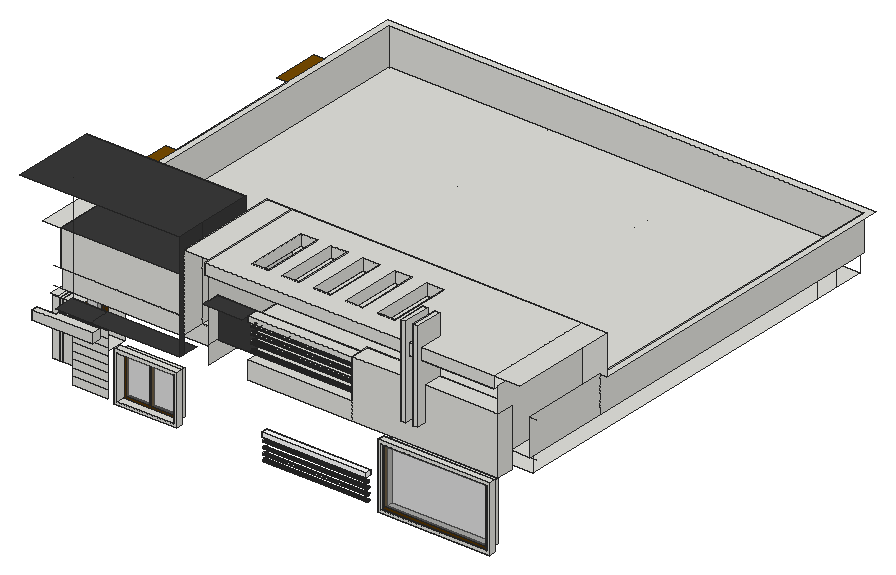
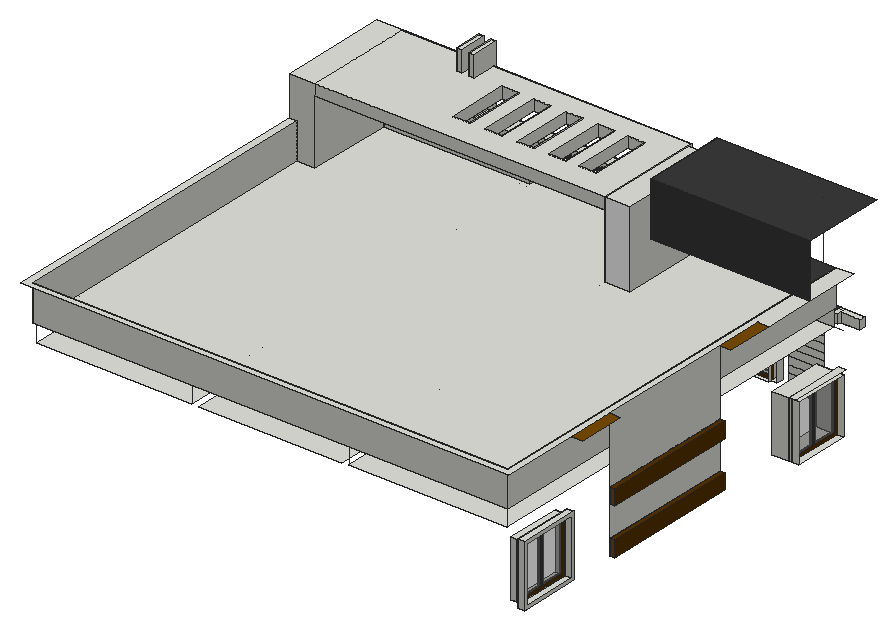
# SketchUp Ruby script. Lengths in inches.
U = 1.inch
M = Sketchup.active_model
def pt(a) = Geom::Point3d.new(a.map { |v| v * U })
def face(e, loops, mat)
  f = e.add_face(loops[0].map { |a| pt(a) })
  loops[1..].each { |l| e.add_face(l.map { |a| pt(a) }).erase! }
  f.material = f.back_material = mat if mat
  f
end
# faces: each face lists its corners as indices into pts; further lists are holes
def faces(e, pts, list, mat = nil) = list.each { |f| face(e, (f[0].is_a?(Array) ? f : [f]).map { |l| l.map { |i| pts[i] } }, mat) }
# xy, xz, yz: faces in a plane at the given z, y or x. An outline is a flat list of corners, or four numbers for a rectangle; further outlines are holes
def ring(l) = l.size == 4 ? [[l[0], l[1]], [l[2], l[1]], [l[2], l[3]], [l[0], l[3]]] : l.each_slice(2).to_a
def flat(e, list, mat, &to3) = list.each { |f| face(e, (f[0].is_a?(Array) ? f : [f]).map { |l| ring(l).map { |u, v| to3.(u, v) } }, mat) }
def xy(e, z, list, mat = nil) = flat(e, list, mat) { |x, y| [x, y, z] }
def xz(e, y, list, mat = nil) = flat(e, list, mat) { |x, z| [x, y, z] }
def yz(e, x, list, mat = nil) = flat(e, list, mat) { |y, z| [x, y, z] }
def lines(e, pts, list) = list.each { |a, b| e.add_line(pt(pts[a]), pt(pts[b])) }
# prism: a flat outline (further loops are holes) pulled along v
def prism(e, loops, v, mat = nil)
  f = face(e, loops, mat); d = Geom::Vector3d.new(v.map { |x| x * U })
  f.pushpull(f.normal.samedirection?(d) ? d.length : -d.length)
end
def box(e, o, s, mat = nil) = prism(e, [[o, [o[0] + s[0], o[1], o[2]], [o[0] + s[0], o[1] + s[1], o[2]], [o[0], o[1] + s[1], o[2]]]], [0, 0, s[2]], mat)
def at(x, y, z, deg = 0) = Geom::Transformation.translation(pt([x, y, z])) * Geom::Transformation.rotation(ORIGIN, Z_AXIS, deg.degrees)
def axes(o, x, y, z) = Geom::Transformation.new([*x, 0, *y, 0, *z, 0, *pt(o).to_a, 1])
def part(name) = M.definitions.add(name)
# library, detail: a bought-in or finely detailed component or shape, given as its bounding box
def library(name, o, s) = part(name).tap { |d| box(d.entities, o, s) }
def detail(e, o, s) = box(e.add_group.entities, o, s)
def put(e, d, t, mat = nil) = e.add_instance(d, t).tap { |i| i.material = mat if mat }
def group(e, t, mat = nil) = e.add_group.tap { |g| g.transformation = t; g.material = mat if mat }.entities
root = M.entities
M.materials.add("[Color C07]").color = [120, 76, 0]
M.materials.add("[Color C08]").color = [85, 51, 0]
M.materials.add("[Color M00]").color = [255, 255, 255]
M.materials.add("[Color M07]").color = [58, 58, 58]
M.materials.add("[Translucent Glass Gray]").color = [128, 128, 128]
M.materials["[Translucent Glass Gray]"].alpha = 0.5
M.materials.add("[Wood Veneer 01]1").color = [120, 70, 37]
c1 = part("Group\#4")
xy(c1.entities,0,[[0,0,0.4375,8.25]],"[Color C08]")
xy(c1.entities,9.875,[[0,0,0.4375,8.25]],"[Color C08]")
xz(c1.entities,0,[[0,0,0.4375,9.875]],"[Color C08]")
xz(c1.entities,0.45,[[0,0.45,0.4375,9.42]],"[Color C08]")
xz(c1.entities,4.05,[[0,0.49,0.4375,9.45]],"[Color C08]")
xz(c1.entities,4.38,[[0,0.49,0.4375,9.45]],"[Color C08]")
xz(c1.entities,7.8,[[0,0.45,0.4375,9.42]],"[Color C08]")
xz(c1.entities,8.25,[[0,0,0.4375,9.875]],"[Color C08]")
yz(c1.entities,0,[[[0,0,8.25,9.875],[0.45,0.45,4.05,0.49,4.05,9.45,0.45,9.42],[7.8,0.45,7.8,9.42,4.38,9.45,4.38,0.49]]],"[Color C08]")
yz(c1.entities,0,[[0.45,0.45,0.45,9.42,4.05,9.45,4.05,0.49],[7.8,0.45,4.38,0.49,4.38,9.45,7.8,9.42]],"[Translucent Glass Gray]")
yz(c1.entities,0.4375,[[[0,0,8.25,9.875],[0.45,0.45,0.45,9.42,4.05,9.45,4.05,0.49],[7.8,0.45,4.38,0.49,4.38,9.45,7.8,9.42]]],"[Color C08]")
p = [[0,4.05,0.49],[0,0.45,0.45],[0.4375,0.45,0.45],[0.4375,4.05,0.49],[0,7.8,0.45],[0,4.38,0.49],
  [0.4375,4.38,0.49],[0.4375,7.8,0.45],[0,0.45,9.42],[0,4.05,9.45],[0.4375,4.05,9.45],[0.4375,0.45,9.42],
  [0,4.38,9.45],[0,7.8,9.42],[0.4375,7.8,9.42],[0.4375,4.38,9.45]]
faces(c1.entities,p,[[0,1,2,3],[4,5,6,7],[8,9,10,11],[12,13,14,15]],"[Color C08]")
c2 = part("Group\#3")
xy(c2.entities,0,[[0,0,69.125,3.25]],"[Color C08]")
xy(c2.entities,1.72,[[1.72,0,67.41,3.25]],"[Color C08]")
xy(c2.entities,48.28,[[1.72,0,67.41,3.25]],"[Color C08]")
xy(c2.entities,50,[[0,0,69.125,3.25]],"[Color C08]")
xz(c2.entities,0,[[[0,0,69.125,50],[1.72,1.72,67.41,48.28]]],"[Color C08]")
xz(c2.entities,0,[[1.72,1.72,67.41,48.28]],"[Translucent Glass Gray]")
xz(c2.entities,3.25,[[[0,0,69.125,50],[1.72,1.72,67.41,48.28]]],"[Color C08]")
yz(c2.entities,0,[[0,0,3.25,50]],"[Color C08]")
yz(c2.entities,1.72,[[0,1.72,3.25,48.28]],"[Color C08]")
yz(c2.entities,67.41,[[0,1.72,3.25,48.28]],"[Color C08]")
yz(c2.entities,69.125,[[0,0,3.25,50]],"[Color C08]")
prism(root,[[[70.87,180.75,670.36],[95.94,180.75,670.36],[95.94,185.5,670.36],[151.38,185.5,670.36],[151.38,172.6875,670.36],[70.87,172.6875,670.36]]],[0,0,12.45])
prism(root,[[[347.125,192.875,732.3],[347.125,193.13,732.92],[347.125,193.54,733.45],[347.125,194.07,733.86],[347.125,194.6875,734.12],[347.125,195.35,734.2],[347.125,196.01,734.12],[347.125,196.63,733.86],[347.125,197.16,733.45],[347.125,197.57,732.92],[347.125,197.83,732.3],[347.125,197.91,731.64],[347.125,197.83,730.98],[347.125,197.57,730.36],[347.125,197.16,729.83],[347.125,196.63,729.42],[347.125,196.01,729.17],[347.125,195.35,729.08],[347.125,194.6875,729.17],[347.125,194.07,729.42],[347.125,193.54,729.83],[347.125,193.13,730.36],[347.125,192.875,730.98],[347.125,192.79,731.64]]],[138.875,0,0])
xy(root,581.63,[[39.625,246.5625,48.625,321.8125],[48.625,246.5625,75,321.8125]])
xy(root,583.28,[[510.53,200.375,659.59,209.375]])
xy(root,587.28,[[514.53,200.375,655.59,209.375],[514.53,209.375,655.59,218.375]])
xy(root,588.78,[[158.4,200.375,241.77,209.375]])
xy(root,590.06,[[56.4375,423.72,63,608.17]],"[Color C08]")
xy(root,592.78,[[162.4,200.375,237.77,218.375]])
xy(root,595.54,[[54,679.03,63,761.4]])
xy(root,599.54,[[54,683.03,63,757.4],[63,683.03,75,757.4]])
xy(root,611.09,[[347.125,210.1875,486.25,218.5625]],"[Color M00]")
xy(root,611.45,[[56.4375,423.72,63,608.17]],"[Color C08]")
xy(root,617,[[347.125,210.1875,486.25,218.5625]],"[Color M00]")
xy(root,650.97,[[162.4,200.375,237.77,218.375]])
xy(root,651.9375,[[56.4375,423.72,63,608.17]],"[Color C08]")
xy(root,654.97,[[158.4,200.375,241.77,209.375]])
xy(root,656.88,[[39.625,246.5625,48.625,321.8125],[48.625,246.5625,75,321.8125]])
xy(root,660.88,[[39.625,242.5625,48.625,325.8125]])
xy(root,666.09,[[514.53,200.375,655.59,209.375],[514.53,209.375,655.59,218.375]])
xy(root,668.5625,[[338.07,326.375,453.82,335.375]])
xy(root,670.09,[[510.53,200.375,659.59,209.375]])
xy(root,673.33,[[56.4375,423.72,63,608.17]],"[Color C08]")
xy(root,673.91,[[54,683.03,63,757.4],[63,683.03,75,757.4]])
xy(root,677.91,[[54,679.03,63,761.4]])
xy(root,689,[[347.125,187.375,347.125,237.56,295.1875,237.56,295.1875,326.375,486.25,326.375,486.25,187.375],[486.25,187.375,681.47,209.375],[75,218.375,286.1875,764.25],[495.25,218.375,703.3125,764.25],[295.1875,335.375,486.25,764.25]])
xy(root,689,[[95.94,180.75,143.14,209.375],[143.14,180.75,261.34,209.375]],"[Color M07]")
xy(root,713,[[347.125,187.375,486.25,201.8125],[295.1875,201.8125,486.25,201.8125,486.25,212.5625,681.47,212.5625,681.47,326.375,706.3125,326.375,706.3125,767.25,72,767.25,72,218.375,261.34,218.375,261.34,326.375,295.1875,326.375],[681.47,209.375,706.3125,326.375],[261.34,218.375,286.1875,326.375]])
xy(root,720.5625,[[560.32,175.625,566.88,187.375],[576.82,175.625,583.38,187.375]])
xy(root,758.77,[[347.125,187.375,486.25,201.8125]])
xy(root,761,[[48.625,218.375,72,291.52],[48.625,291.52,72,291.52,72,767.25,706.3125,767.25,706.3125,326.375,715.3125,326.375,715.3125,776.25,63,776.25,63,360.49,48.625,360.49]])
xy(root,761,[[48.625,360.49,63,423.72],[48.625,608.17,63,671.4]],"[Color C07]")
xy(root,761,[[72,218.375,261.3125,291.52]],"[Color M07]")
xy(root,766,[[347.125,187.375,486.25,201.8125],[486.25,187.375,560.32,212.5625],[560.32,187.375,566.88,212.5625],[566.88,187.375,576.82,212.5625],[576.82,187.375,583.38,212.5625],
  [583.38,187.375,681.47,212.5625]])
xy(root,766,[[295.1875,177.125,347.125,201.8125]],"[Color M07]")
xy(root,799.39,[[[295.1875,180.75,681.47,326.375],[334.41,209.27,357.09,291.34],[375.09,209.27,397.78,291.34],[417.38,208.94,440.07,291.01],[460.38,208.94,483.07,291.01],[503.13,208.94,525.82,291.01]]])
xy(root,814.1875,[[[295.1875,180.75,681.47,326.375],[334.41,209.27,357.09,291.34],[375.09,209.27,397.78,291.34],[417.38,208.94,440.07,291.01],[460.38,208.94,483.07,291.01],[503.13,208.94,525.82,291.01]],[681.47,180.75,715.3125,326.375],[261.34,187.375,295.1875,326.375]])
xy(root,833,[[48.625,180.75,261.34,180.75,261.34,218.375,261.3125,218.375,261.3125,291.52,48.625,291.52]],"[Color M07]")
xy(root,841.5625,[[560.32,175.625,566.88,212.5625],[576.82,175.625,583.38,212.5625]])
xz(root,175.625,[[560.32,720.5625,566.88,841.5625],[576.82,720.5625,583.38,841.5625]])
xz(root,180.75,[[295.1875,799.39,681.47,814.1875]])
xz(root,187.375,[[347.125,689,486.25,713],[486.25,689,681.47,689,681.47,766,583.38,766,583.38,720.5625,576.82,720.5625,576.82,766,566.88,766,566.88,720.5625,560.32,720.5625,560.32,766,486.25,766],[560.32,720.5625,566.88,766],[576.82,720.5625,583.38,766],[347.125,758.77,486.25,766]])
xz(root,200.375,[[[510.53,583.28,659.59,670.09],[514.53,587.28,655.59,666.09]],[[158.4,588.78,241.77,654.97],[162.4,592.78,237.77,650.97]]])
xz(root,201.8125,[[347.125,758.77,486.25,766]])
xz(root,201.8125,[[295.1875,713,347.125,766]],"[Color M07]")
xz(root,208.94,[[417.38,799.39,440.07,814.1875],[460.38,799.39,483.07,814.1875],[503.13,799.39,525.82,814.1875]])
xz(root,209.27,[[334.41,799.39,357.09,814.1875],[375.09,799.39,397.78,814.1875]])
xz(root,209.375,[[[510.53,583.28,659.59,670.09],[514.53,587.28,655.59,666.09]],[95.94,585.52,143.14,595.71],[95.94,595.71,143.14,605.9],[95.94,605.9,143.14,616.09],[95.94,616.09,143.14,626.27],
  [95.94,626.27,143.14,636.46],[95.94,636.46,143.14,646.65],[95.94,646.65,143.14,656.84],[95.94,656.84,143.14,667.02],[95.94,667.02,143.14,677.21],
  [95.94,677.21,143.14,689]])
xz(root,210.1875,[[347.125,611.09,486.25,617]],"[Color M00]")
xz(root,212.5625,[[486.25,713,681.47,766],[560.32,766,566.88,841.5625],[576.82,766,583.38,841.5625]])
xz(root,218.375,[[75,689,286.1875,713],[72,713,72,761,261.3125,761,261.3125,833,261.34,833,261.34,713]])
xz(root,218.5625,[[347.125,611.09,486.25,617]],"[Color M00]")
xz(root,246.5625,[[39.625,581.63,48.625,656.88],[48.625,581.63,75,656.88]])
xz(root,291.01,[[417.38,799.39,440.07,814.1875],[460.38,799.39,483.07,814.1875],[503.13,799.39,525.82,814.1875]])
xz(root,291.34,[[334.41,799.39,357.09,814.1875],[375.09,799.39,397.78,814.1875]])
xz(root,291.52,[[48.625,761,261.3125,833]],"[Color M07]")
xz(root,321.8125,[[39.625,581.63,48.625,656.88],[48.625,581.63,75,656.88]])
xz(root,326.375,[[681.47,713,681.47,814.1875,715.3125,814.1875,715.3125,761,706.3125,761,706.3125,713],[295.1875,799.39,681.47,814.1875]])
xz(root,326.375,[[261.34,713,295.1875,814.1875]],"[Color M00]")
xz(root,423.72,[[56.4375,590.06,63,611.45],[56.4375,651.9375,63,673.33]],"[Wood Veneer 01]1")
xz(root,608.17,[[56.4375,590.06,63,611.45],[56.4375,651.9375,63,673.33]],"[Wood Veneer 01]1")
xz(root,679.03,[[54,595.54,63,677.91]])
xz(root,683.03,[[54,599.54,63,673.91],[63,599.54,75,673.91]])
xz(root,757.4,[[54,599.54,63,673.91],[63,599.54,75,673.91]])
xz(root,761.4,[[54,595.54,63,677.91]])
xz(root,767.25,[[72,713,706.3125,761]])
yz(root,54,[[[679.03,595.54,761.4,677.91],[683.03,599.54,757.4,673.91]]])
yz(root,56.4375,[[423.72,590.06,608.17,611.45],[423.72,651.9375,608.17,673.33]],"[Color C08]")
yz(root,63,[[[679.03,595.54,761.4,677.91],[683.03,599.54,757.4,673.91]],[423.72,611.45,608.17,651.9375],[423.72,673.33,608.17,761]])
yz(root,63,[[423.72,590.06,608.17,611.45],[423.72,651.9375,608.17,673.33]],"[Wood Veneer 01]1")
yz(root,72,[[218.375,713,767.25,761]])
yz(root,158.4,[[200.375,588.78,209.375,654.97]])
yz(root,162.4,[[200.375,592.78,218.375,650.97]])
yz(root,237.77,[[200.375,592.78,218.375,650.97]])
yz(root,241.77,[[200.375,588.78,209.375,654.97]])
yz(root,261.3125,[[218.375,761,291.52,833]],"[Color M07]")
yz(root,261.34,[[187.375,713,218.375,814.1875],[218.375,713,326.375,814.1875]])
yz(root,261.34,[[180.75,689,187.375,689,187.375,814.1875,218.375,814.1875,218.375,833,180.75,833]],"[Color M07]")
yz(root,295.1875,[[187.375,689,326.375,713],[187.375,713,201.8125,766],[201.8125,713,326.375,713,326.375,799.39,187.375,799.39,187.375,766,201.8125,766],[180.75,799.39,187.375,814.1875],[187.375,799.39,326.375,814.1875]])
yz(root,334.41,[[209.27,799.39,291.34,814.1875]])
yz(root,347.125,[[195.35,717.83,194.6875,717.92,194.07,718.17,193.54,718.58,193.13,719.11,192.875,719.73,192.79,720.39,192.875,721.05,193.13,721.67,193.54,722.2,194.07,722.61,194.6875,722.87,195.35,722.95,196.01,722.87,196.63,722.61,197.16,722.2,197.57,721.67,197.83,721.05,197.91,720.39,197.83,719.73,197.57,719.11,197.16,718.58,196.63,718.17,196.01,717.92],[195.35,739.2,194.6875,739.29,194.07,739.55,193.54,739.95,193.13,740.48,192.875,741.1,192.79,741.77,192.875,742.43,193.13,743.05,193.54,743.58,194.07,743.98,194.6875,744.24,195.35,744.33,196.01,744.24,196.63,743.98,197.16,743.58,197.57,743.05,197.83,742.43,197.91,741.77,197.83,741.1,197.57,740.48,197.16,739.95,196.63,739.55,196.01,739.29],[195.35,748.77,194.6875,748.85,194.07,749.11,193.54,749.52,193.13,750.05,192.875,750.66,192.79,751.33,192.875,751.99,193.13,752.61,193.54,753.14,194.07,753.55,194.6875,753.8,195.35,753.89,196.01,753.8,196.63,753.55,197.16,753.14,197.57,752.61,197.83,751.99,197.91,751.33,197.83,750.66,197.57,750.05,197.16,749.52,196.63,749.11,196.01,748.85],[187.375,758.77,201.8125,766]])
yz(root,347.125,[[214.58,579.9,214.13,579.96,213.71,580.13,213.35,580.41,213.07,580.77,212.89,581.19,212.83,581.65,212.89,582.1,213.07,582.52,213.35,582.88,213.71,583.16,214.13,583.34,214.58,583.4,215.04,583.34,215.46,583.16,215.82,582.88,216.1,582.52,216.28,582.1,216.33,581.65,216.28,581.19,216.1,580.77,215.82,580.41,215.46,580.13,215.04,579.96],[214.58,587.58,214.13,587.64,213.71,587.82,213.35,588.1,213.07,588.46,212.89,588.88,212.83,589.33,212.89,589.79,213.07,590.21,213.35,590.57,213.71,590.85,214.13,591.03,214.58,591.08,215.04,591.03,215.46,590.85,215.82,590.57,216.1,590.21,216.28,589.79,216.33,589.33,216.28,588.88,216.1,588.46,215.82,588.1,215.46,587.82,215.04,587.64],[214.58,595.15,214.13,595.21,213.71,595.38,213.35,595.66,213.07,596.02,212.89,596.44,212.83,596.9,212.89,597.35,213.07,597.77,213.35,598.13,213.71,598.41,214.13,598.59,214.58,598.65,215.04,598.59,215.46,598.41,215.82,598.13,216.1,597.77,216.28,597.35,216.33,596.9,216.28,596.44,216.1,596.02,215.82,595.66,215.46,595.38,215.04,595.21],[214.41,603.03,213.95,603.09,213.53,603.26,213.17,603.54,212.89,603.9,212.72,604.32,212.66,604.78,212.72,605.23,212.89,605.65,213.17,606.02,213.53,606.29,213.95,606.47,214.41,606.53,214.86,606.47,215.28,606.29,215.64,606.02,215.92,605.65,216.1,605.23,216.16,604.78,216.1,604.32,215.92,603.9,215.64,603.54,215.28,603.26,214.86,603.09],[210.1875,611.09,218.5625,617]],"[Color M00]")
yz(root,357.09,[[209.27,799.39,291.34,814.1875]])
yz(root,375.09,[[209.27,799.39,291.34,814.1875]])
yz(root,397.78,[[209.27,799.39,291.34,814.1875]])
yz(root,417.38,[[208.94,799.39,291.01,814.1875]])
yz(root,440.07,[[208.94,799.39,291.01,814.1875]])
yz(root,460.38,[[208.94,799.39,291.01,814.1875]])
yz(root,483.07,[[208.94,799.39,291.01,814.1875]])
yz(root,486.25,[[218.375,611.09,218.5625,617],[[187.375,713,187.375,758.77,201.8125,758.77,201.8125,766,212.5625,766,212.5625,713],[195.35,717.83,196.01,717.92,196.63,718.17,197.16,718.58,197.57,719.11,197.83,719.73,197.91,720.39,197.83,721.05,197.57,721.67,197.16,722.2,196.63,722.61,196.01,722.87,195.35,722.95,194.6875,722.87,194.07,722.61,193.54,722.2,193.13,721.67,192.875,721.05,192.79,720.39,192.875,719.73,193.13,719.11,193.54,718.58,194.07,718.17,194.6875,717.92],[195.35,739.2,196.01,739.29,196.63,739.55,197.16,739.95,197.57,740.48,197.83,741.1,197.91,741.77,197.83,742.43,197.57,743.05,197.16,743.58,196.63,743.98,196.01,744.24,195.35,744.33,194.6875,744.24,194.07,743.98,193.54,743.58,193.13,743.05,192.875,742.43,192.79,741.77,192.875,741.1,193.13,740.48,193.54,739.95,194.07,739.55,194.6875,739.29],[195.35,748.77,196.01,748.85,196.63,749.11,197.16,749.52,197.57,750.05,197.83,750.66,197.91,751.33,197.83,751.99,197.57,752.61,197.16,753.14,196.63,753.55,196.01,753.8,195.35,753.89,194.6875,753.8,194.07,753.55,193.54,753.14,193.13,752.61,192.875,751.99,192.79,751.33,192.875,750.66,193.13,750.05,193.54,749.52,194.07,749.11,194.6875,748.85]],[187.375,758.77,201.8125,766]])
yz(root,486.25,[[210.1875,611.09,218.375,617]],"[Color M00]")
yz(root,503.13,[[208.94,799.39,291.01,814.1875]])
yz(root,510.53,[[200.375,583.28,209.375,670.09]])
yz(root,514.53,[[200.375,587.28,209.375,666.09],[209.375,587.28,218.375,666.09]])
yz(root,525.82,[[208.94,799.39,291.01,814.1875]])
yz(root,560.32,[[175.625,720.5625,175.625,841.5625,212.5625,841.5625,212.5625,766,187.375,766,187.375,720.5625]])
yz(root,566.88,[[175.625,720.5625,187.375,720.5625,187.375,766,212.5625,766,212.5625,841.5625,175.625,841.5625]])
yz(root,576.82,[[175.625,720.5625,175.625,841.5625,212.5625,841.5625,212.5625,766,187.375,766,187.375,720.5625]])
yz(root,583.38,[[175.625,720.5625,187.375,720.5625,187.375,766,212.5625,766,212.5625,841.5625,175.625,841.5625]])
yz(root,655.59,[[200.375,587.28,209.375,666.09],[209.375,587.28,218.375,666.09]])
yz(root,659.59,[[200.375,583.28,209.375,670.09]])
yz(root,681.47,[[187.375,689,209.375,766],[212.5625,713,212.5625,766,187.375,766,187.375,799.39,326.375,799.39,326.375,713],[209.375,713,212.5625,766]])
yz(root,706.3125,[[209.375,713,326.375,761],[326.375,713,767.25,761]])
p = [[347.125,214.13,579.96],[347.125,214.58,579.9],[486.25,214.58,579.9],[486.25,214.13,579.96],[347.125,215.04,579.96],[486.25,215.04,579.96],
  [347.125,213.71,580.13],[486.25,213.71,580.13],[347.125,215.46,580.13],[486.25,215.46,580.13],[347.125,213.35,580.41],[486.25,213.35,580.41],
  [347.125,215.82,580.41],[486.25,215.82,580.41],[347.125,213.07,580.77],[486.25,213.07,580.77],[347.125,216.1,580.77],[486.25,216.1,580.77],
  [347.125,212.89,581.19],[486.25,212.89,581.19],[347.125,216.28,581.19],[486.25,216.28,581.19],[347.125,212.83,581.65],[486.25,212.83,581.65],
  [347.125,216.33,581.65],[486.25,216.33,581.65],[347.125,212.89,582.1],[486.25,212.89,582.1],[347.125,216.28,582.1],[486.25,216.28,582.1],
  [347.125,213.07,582.52],[486.25,213.07,582.52],[347.125,216.1,582.52],[486.25,216.1,582.52],[347.125,213.35,582.88],[486.25,213.35,582.88],
  [347.125,215.82,582.88],[486.25,215.82,582.88],[347.125,213.71,583.16],[486.25,213.71,583.16],[347.125,215.46,583.16],[486.25,215.46,583.16],
  [347.125,214.13,583.34],[486.25,214.13,583.34],[347.125,215.04,583.34],[486.25,215.04,583.34],[347.125,214.58,583.4],[486.25,214.58,583.4],
  [347.125,213.71,587.82],[347.125,214.13,587.64],[486.25,214.13,587.64],[486.25,213.71,587.82],[347.125,214.58,587.58],[486.25,214.58,587.58],
  [347.125,215.04,587.64],[486.25,215.04,587.64],[347.125,215.46,587.82],[486.25,215.46,587.82],[347.125,213.35,588.1],[486.25,213.35,588.1],
  [347.125,215.82,588.1],[486.25,215.82,588.1],[347.125,213.07,588.46],[486.25,213.07,588.46],[347.125,216.1,588.46],[486.25,216.1,588.46],
  [347.125,212.89,588.88],[486.25,212.89,588.88],[347.125,216.28,588.88],[486.25,216.28,588.88],[347.125,212.83,589.33],[486.25,212.83,589.33],
  [347.125,216.33,589.33],[486.25,216.33,589.33],[347.125,212.89,589.79],[486.25,212.89,589.79],[347.125,216.28,589.79],[486.25,216.28,589.79],
  [347.125,213.07,590.21],[486.25,213.07,590.21],[347.125,216.1,590.21],[486.25,216.1,590.21],[347.125,213.35,590.57],[486.25,213.35,590.57],
  [347.125,215.82,590.57],[486.25,215.82,590.57],[347.125,213.71,590.85],[486.25,213.71,590.85],[347.125,215.46,590.85],[486.25,215.46,590.85],
  [347.125,214.13,591.03],[486.25,214.13,591.03],[347.125,215.04,591.03],[486.25,215.04,591.03],[347.125,214.58,591.08],[486.25,214.58,591.08],
  [347.125,214.13,595.21],[347.125,214.58,595.15],[486.25,214.58,595.15],[486.25,214.13,595.21],[347.125,215.04,595.21],[486.25,215.04,595.21],
  [347.125,213.71,595.38],[486.25,213.71,595.38],[347.125,215.46,595.38],[486.25,215.46,595.38],[347.125,213.35,595.66],[486.25,213.35,595.66],
  [347.125,215.82,595.66],[486.25,215.82,595.66],[347.125,213.07,596.02],[486.25,213.07,596.02],[347.125,216.1,596.02],[486.25,216.1,596.02],
  [347.125,212.89,596.44],[486.25,212.89,596.44],[347.125,216.28,596.44],[486.25,216.28,596.44],[347.125,212.83,596.9],[486.25,212.83,596.9],
  [347.125,216.33,596.9],[486.25,216.33,596.9],[347.125,212.89,597.35],[486.25,212.89,597.35],[347.125,216.28,597.35],[486.25,216.28,597.35],
  [347.125,213.07,597.77],[486.25,213.07,597.77],[347.125,216.1,597.77],[486.25,216.1,597.77],[347.125,213.35,598.13],[486.25,213.35,598.13],
  [347.125,215.82,598.13],[486.25,215.82,598.13],[347.125,213.71,598.41],[486.25,213.71,598.41],[347.125,215.46,598.41],[486.25,215.46,598.41],
  [347.125,214.13,598.59],[486.25,214.13,598.59],[347.125,215.04,598.59],[486.25,215.04,598.59],[347.125,214.58,598.65],[486.25,214.58,598.65],
  [347.125,213.95,603.09],[347.125,214.41,603.03],[486.25,214.41,603.03],[486.25,213.95,603.09],[347.125,214.86,603.09],[486.25,214.86,603.09],
  [347.125,213.53,603.26],[486.25,213.53,603.26],[347.125,215.28,603.26],[486.25,215.28,603.26],[347.125,213.17,603.54],[486.25,213.17,603.54],
  [347.125,215.64,603.54],[486.25,215.64,603.54],[347.125,212.89,603.9],[486.25,212.89,603.9],[347.125,215.92,603.9],[486.25,215.92,603.9],
  [347.125,212.72,604.32],[486.25,212.72,604.32],[347.125,216.1,604.32],[486.25,216.1,604.32],[347.125,212.66,604.78],[486.25,212.66,604.78],
  [347.125,216.16,604.78],[486.25,216.16,604.78],[347.125,212.72,605.23],[486.25,212.72,605.23],[347.125,216.1,605.23],[486.25,216.1,605.23],
  [347.125,212.89,605.65],[486.25,212.89,605.65],[347.125,215.92,605.65],[486.25,215.92,605.65],[347.125,213.17,606.02],[486.25,213.17,606.02],
  [347.125,215.64,606.02],[486.25,215.64,606.02],[347.125,213.53,606.29],[486.25,213.53,606.29],[347.125,215.28,606.29],[486.25,215.28,606.29],
  [347.125,213.95,606.47],[486.25,213.95,606.47],[347.125,214.86,606.47],[486.25,214.86,606.47],[347.125,214.41,606.53],[486.25,214.41,606.53],
  [347.125,194.6875,717.92],[347.125,195.35,717.83],[486.25,195.35,717.83],[486.25,194.6875,717.92],[347.125,196.01,717.92],[486.25,196.01,717.92],
  [347.125,194.07,718.17],[486.25,194.07,718.17],[347.125,196.63,718.17],[486.25,196.63,718.17],[347.125,193.54,718.58],[486.25,193.54,718.58],
  [347.125,197.16,718.58],[486.25,197.16,718.58],[347.125,193.13,719.11],[486.25,193.13,719.11],[347.125,197.57,719.11],[486.25,197.57,719.11],
  [347.125,192.875,719.73],[486.25,192.875,719.73],[347.125,197.83,719.73],[486.25,197.83,719.73],[347.125,192.79,720.39],[486.25,192.79,720.39],
  [347.125,197.91,720.39],[486.25,197.91,720.39],[347.125,192.875,721.05],[486.25,192.875,721.05],[347.125,197.83,721.05],[486.25,197.83,721.05],
  [347.125,193.13,721.67],[486.25,193.13,721.67],[347.125,197.57,721.67],[486.25,197.57,721.67],[347.125,193.54,722.2],[486.25,193.54,722.2],
  [347.125,197.16,722.2],[486.25,197.16,722.2],[347.125,194.07,722.61],[486.25,194.07,722.61],[347.125,196.63,722.61],[486.25,196.63,722.61],
  [347.125,194.6875,722.87],[486.25,194.6875,722.87],[347.125,196.01,722.87],[486.25,196.01,722.87],[347.125,195.35,722.95],[486.25,195.35,722.95],
  [347.125,194.6875,739.29],[347.125,195.35,739.2],[486.25,195.35,739.2],[486.25,194.6875,739.29],[347.125,196.01,739.29],[486.25,196.01,739.29],
  [347.125,194.07,739.55],[486.25,194.07,739.55],[347.125,196.63,739.55],[486.25,196.63,739.55],[347.125,193.54,739.95],[486.25,193.54,739.95],
  [347.125,197.16,739.95],[486.25,197.16,739.95],[347.125,193.13,740.48],[486.25,193.13,740.48],[347.125,197.57,740.48],[486.25,197.57,740.48],
  [347.125,192.875,741.1],[486.25,192.875,741.1],[347.125,197.83,741.1],[486.25,197.83,741.1],[347.125,192.79,741.77],[486.25,192.79,741.77],
  [347.125,197.91,741.77],[486.25,197.91,741.77],[347.125,192.875,742.43],[486.25,192.875,742.43],[347.125,197.83,742.43],[486.25,197.83,742.43],
  [347.125,193.13,743.05],[486.25,193.13,743.05],[347.125,197.57,743.05],[486.25,197.57,743.05],[347.125,193.54,743.58],[486.25,193.54,743.58],
  [347.125,197.16,743.58],[486.25,197.16,743.58],[347.125,194.07,743.98],[486.25,194.07,743.98],[347.125,196.63,743.98],[486.25,196.63,743.98],
  [347.125,194.6875,744.24],[486.25,194.6875,744.24],[347.125,196.01,744.24],[486.25,196.01,744.24],[347.125,195.35,744.33],[486.25,195.35,744.33],
  [347.125,194.6875,748.85],[347.125,195.35,748.77],[486.25,195.35,748.77],[486.25,194.6875,748.85],[347.125,196.01,748.85],[486.25,196.01,748.85],
  [347.125,194.07,749.11],[486.25,194.07,749.11],[347.125,196.63,749.11],[486.25,196.63,749.11],[347.125,193.54,749.52],[486.25,193.54,749.52],
  [347.125,197.16,749.52],[486.25,197.16,749.52],[347.125,193.13,750.05],[486.25,193.13,750.05],[347.125,197.57,750.05],[486.25,197.57,750.05],
  [347.125,192.875,750.66],[486.25,192.875,750.66],[347.125,197.83,750.66],[486.25,197.83,750.66],[347.125,192.79,751.33],[486.25,192.79,751.33],
  [347.125,197.91,751.33],[486.25,197.91,751.33],[347.125,192.875,751.99],[486.25,192.875,751.99],[347.125,197.83,751.99],[486.25,197.83,751.99],
  [347.125,193.13,752.61],[486.25,193.13,752.61],[347.125,197.57,752.61],[486.25,197.57,752.61],[347.125,193.54,753.14],[486.25,193.54,753.14],
  [347.125,197.16,753.14],[486.25,197.16,753.14],[347.125,194.07,753.55],[486.25,194.07,753.55],[347.125,196.63,753.55],[486.25,196.63,753.55],
  [347.125,194.6875,753.8],[486.25,194.6875,753.8],[347.125,196.01,753.8],[486.25,196.01,753.8],[347.125,195.35,753.89],[486.25,195.35,753.89],
  [486.25,218.375,689],[486.25,218.375,713],[703.3125,764.25,689],[703.3125,764.25,713],[495.25,218.375,689],[495.25,218.375,713],
  [495.25,764.25,689],[495.25,764.25,713],[703.3125,692.16,689],[703.3125,692.16,713],[703.3125,723.91,689],[703.3125,723.91,713],
  [703.3125,218.375,689],[703.3125,218.375,713],[286.1875,612.76,689],[286.1875,612.76,713],[75,764.25,689],[75,764.25,713],
  [286.1875,764.25,689],[286.1875,764.25,713],[486.25,679.79,689],[486.25,679.79,713],[295.1875,335.375,689],[295.1875,335.375,713],
  [486.25,658.92,689],[486.25,658.92,713],[486.25,335.375,689],[486.25,335.375,713],[706.3125,209.375,713],[715.3125,209.375,713],
  [72,218.375,713],[63,218.375,713],[706.3125,209.375,761],[715.3125,209.375,761],[286.1875,218.375,689],[295.1875,218.375,689],
  [75,218.375,689],[63,218.375,689],[95.94,209.375,689],[95.94,209.375,833]]
faces(root,p,[[0,1,2,3],[1,4,5,2],[6,0,3,7],[4,8,9,5],[10,6,7,11],[8,12,13,9],[14,10,11,15],[12,16,17,13],
  [18,14,15,19],[16,20,21,17],[22,18,19,23],[20,24,25,21],[26,22,23,27],[24,28,29,25],[30,26,27,31],[28,32,33,29],
  [34,30,31,35],[32,36,37,33],[38,34,35,39],[36,40,41,37],[42,38,39,43],[40,44,45,41],[46,42,43,47],[44,46,47,45],
  [48,49,50,51],[49,52,53,50],[52,54,55,53],[54,56,57,55],[58,48,51,59],[56,60,61,57],[62,58,59,63],[60,64,65,61],
  [66,62,63,67],[64,68,69,65],[70,66,67,71],[68,72,73,69],[74,70,71,75],[72,76,77,73],[78,74,75,79],[76,80,81,77],
  [82,78,79,83],[80,84,85,81],[86,82,83,87],[84,88,89,85],[90,86,87,91],[88,92,93,89],[94,90,91,95],[92,94,95,93],
  [96,97,98,99],[97,100,101,98],[102,96,99,103],[100,104,105,101],[106,102,103,107],[104,108,109,105],[110,106,107,111],[108,112,113,109],
  [114,110,111,115],[112,116,117,113],[118,114,115,119],[116,120,121,117],[122,118,119,123],[120,124,125,121],[126,122,123,127],[124,128,129,125],
  [130,126,127,131],[128,132,133,129],[134,130,131,135],[132,136,137,133],[138,134,135,139],[136,140,141,137],[142,138,139,143],[140,142,143,141],
  [144,145,146,147],[145,148,149,146],[150,144,147,151],[148,152,153,149],[154,150,151,155],[152,156,157,153],[158,154,155,159],[156,160,161,157],
  [162,158,159,163],[160,164,165,161],[166,162,163,167],[164,168,169,165],[170,166,167,171],[168,172,173,169],[174,170,171,175],[172,176,177,173],
  [178,174,175,179],[176,180,181,177],[182,178,179,183],[180,184,185,181],[186,182,183,187],[184,188,189,185],[190,186,187,191],[188,190,191,189]],"[Color M00]")
faces(root,p,[[192,193,194,195],[193,196,197,194],[198,192,195,199],[196,200,201,197],[202,198,199,203],[200,204,205,201],[206,202,203,207],[204,208,209,205],
  [210,206,207,211],[208,212,213,209],[214,210,211,215],[212,216,217,213],[218,214,215,219],[216,220,221,217],[222,218,219,223],[220,224,225,221],
  [226,222,223,227],[224,228,229,225],[230,226,227,231],[228,232,233,229],[234,230,231,235],[232,236,237,233],[238,234,235,239],[236,238,239,237],
  [240,241,242,243],[241,244,245,242],[246,240,243,247],[244,248,249,245],[250,246,247,251],[248,252,253,249],[254,250,251,255],[252,256,257,253],
  [258,254,255,259],[256,260,261,257],[262,258,259,263],[260,264,265,261],[266,262,263,267],[264,268,269,265],[270,266,267,271],[268,272,273,269],
  [274,270,271,275],[272,276,277,273],[278,274,275,279],[276,280,281,277],[282,278,279,283],[280,284,285,281],[286,282,283,287],[284,286,287,285],
  [288,289,290,291],[289,292,293,290],[294,288,291,295],[292,296,297,293],[298,294,295,299],[296,300,301,297],[302,298,299,303],[300,304,305,301],
  [306,302,303,307],[304,308,309,305],[310,306,307,311],[308,312,313,309],[314,310,311,315],[312,316,317,313],[318,314,315,319],[316,320,321,317],
  [322,318,319,323],[320,324,325,321],[326,322,323,327],[324,328,329,325],[330,326,327,331],[328,332,333,329],[334,330,331,335],[332,334,335,333]])
lines(root,p,[[336,337],[338,339],[340,341],[342,343],[344,345],[346,347],[348,349],[350,351],[352,353],[354,355],[356,357],[358,359],
  [360,361],[362,363],[364,365],[366,367],[368,369],[370,371],[372,373],[374,375]])
put(root,c1,axes([48.625,246.5625,581.63],[8.6376,0,0],[0,9.1053,0],[0,0,7.62025]))
put(root,c2,axes([514.53,202.875,587.28],[2.04069,0,0],[0,1,0],[0,0,1.57625]))
put(root,c1,axes([237.77,210.51,592.78],[0,6.04632,0],[-9.13636,0,0],[0,0,5.89241]))
put(root,c1,axes([63,683.03,599.54],[8.6376,0,0],[0,9.01515,0],[0,0,7.53165]))
